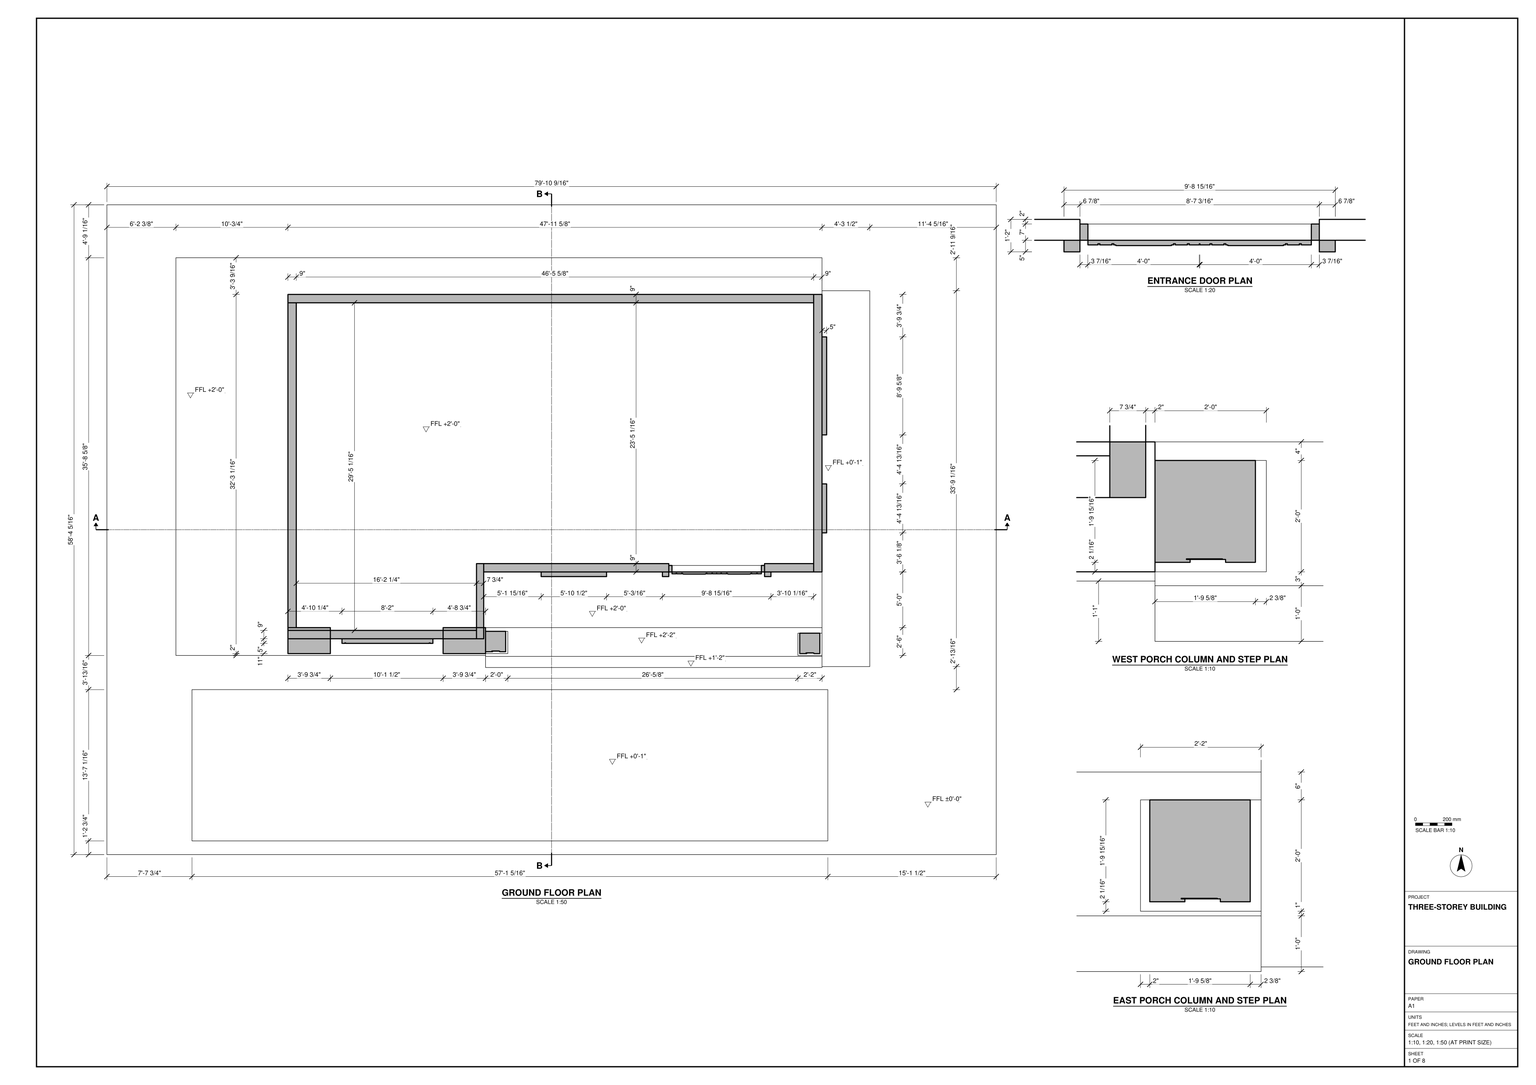
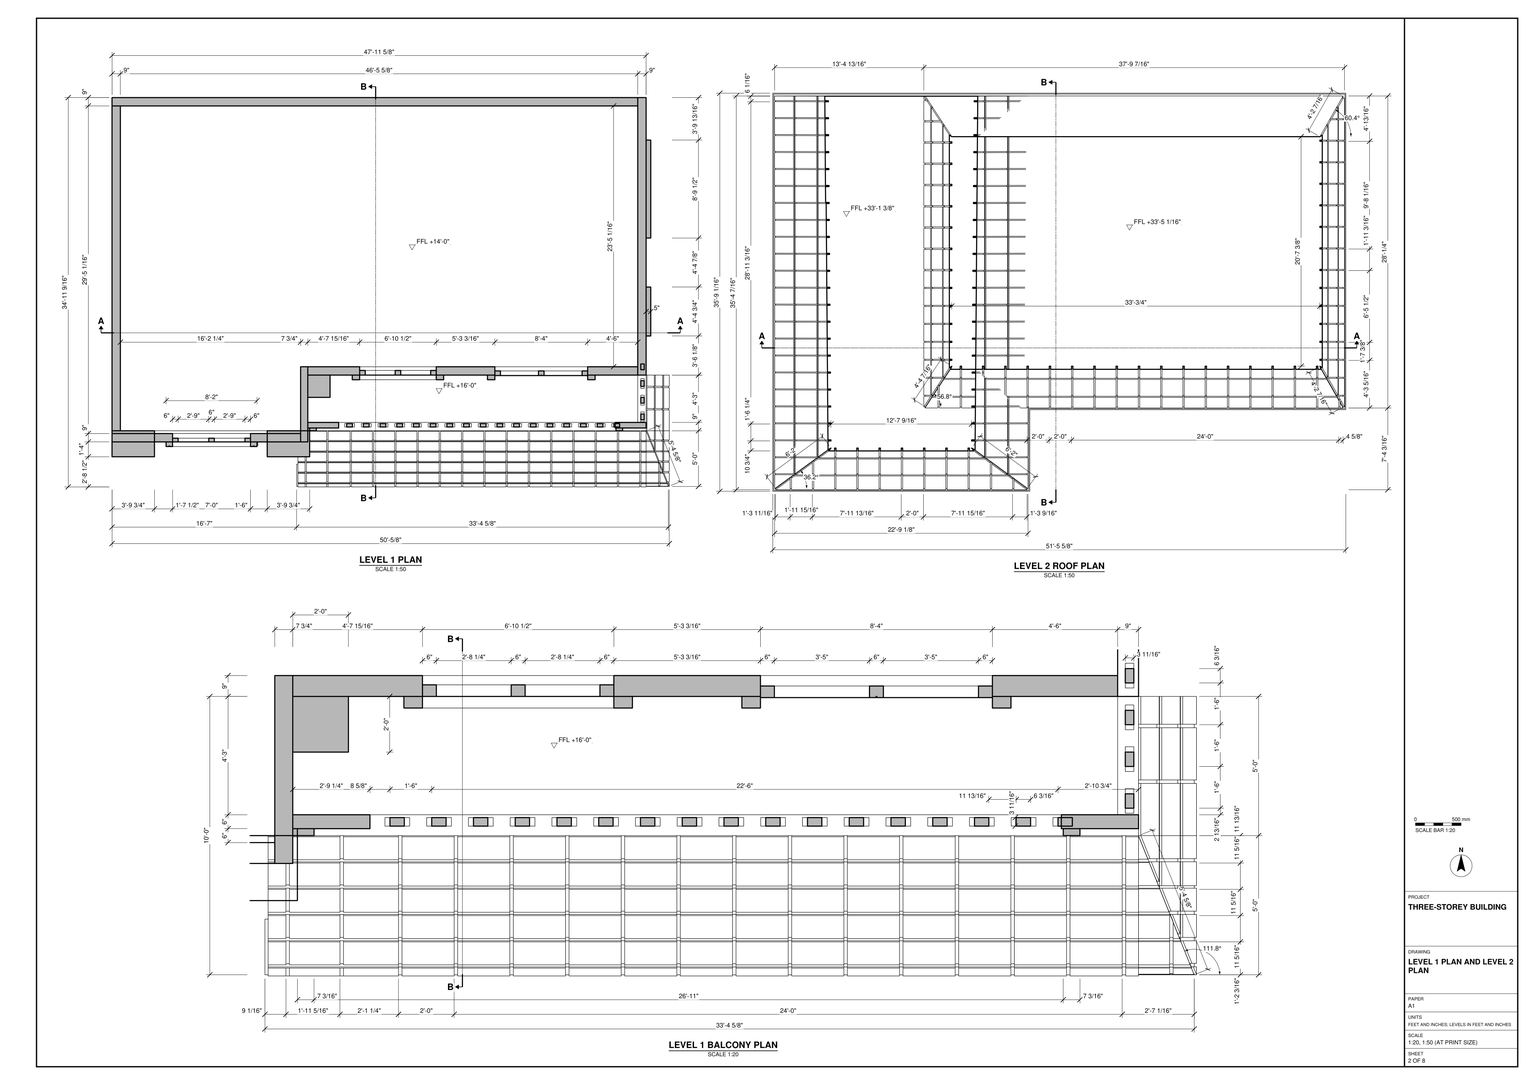
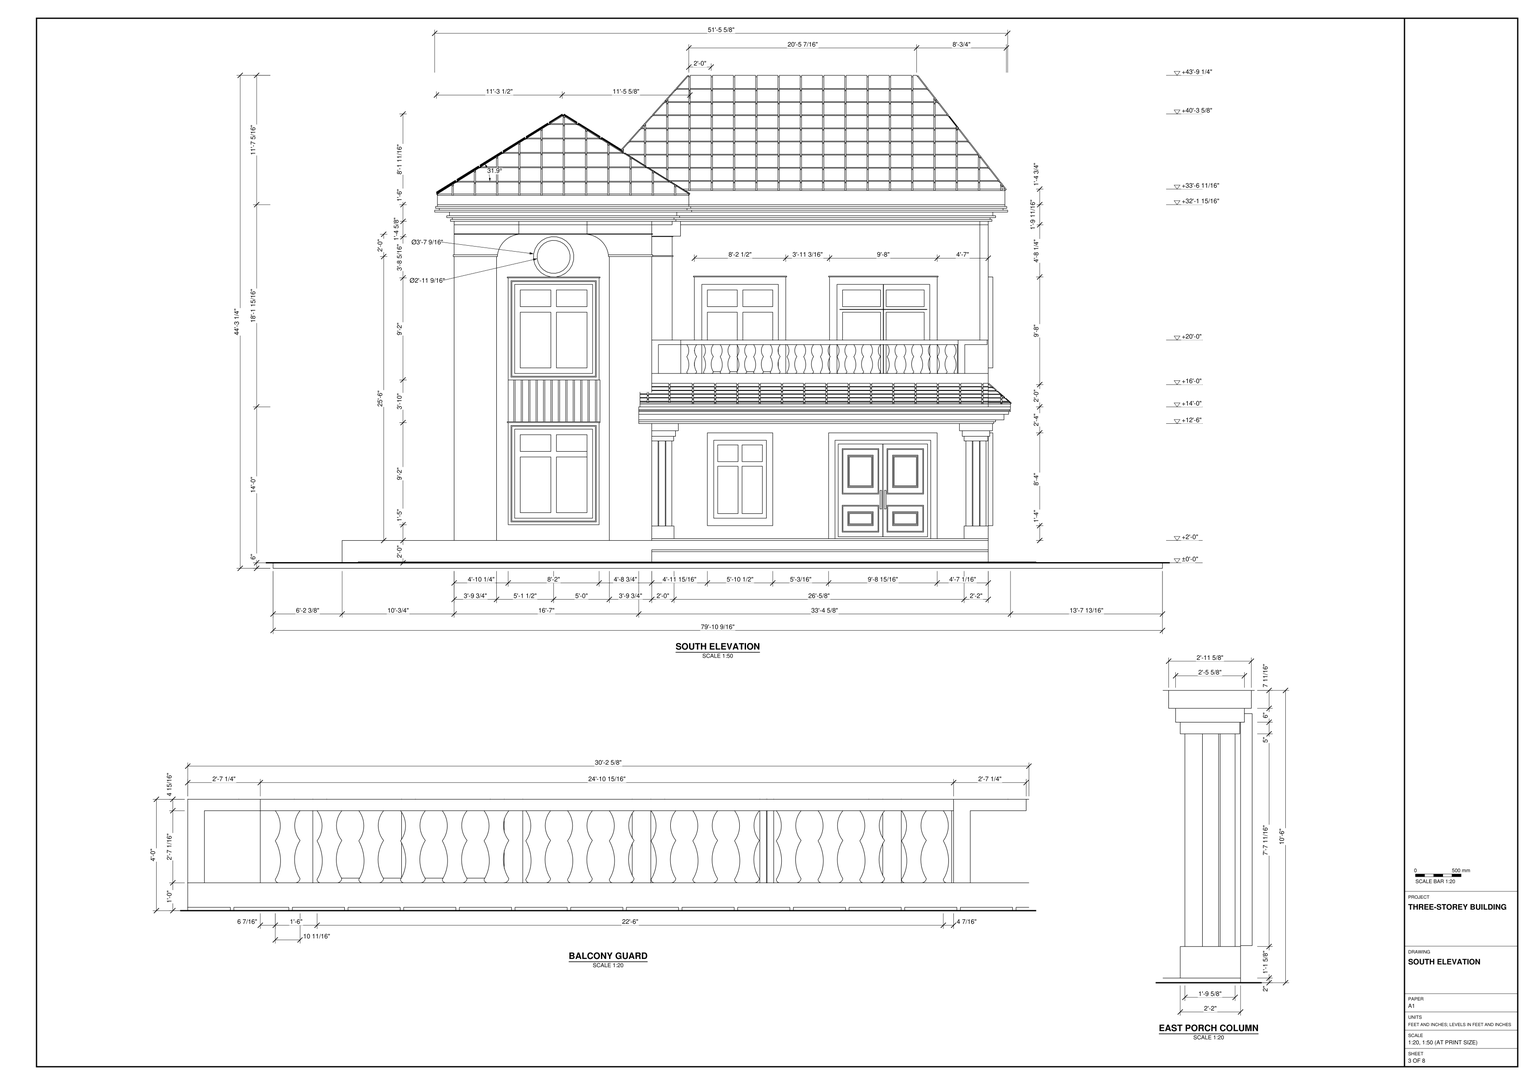
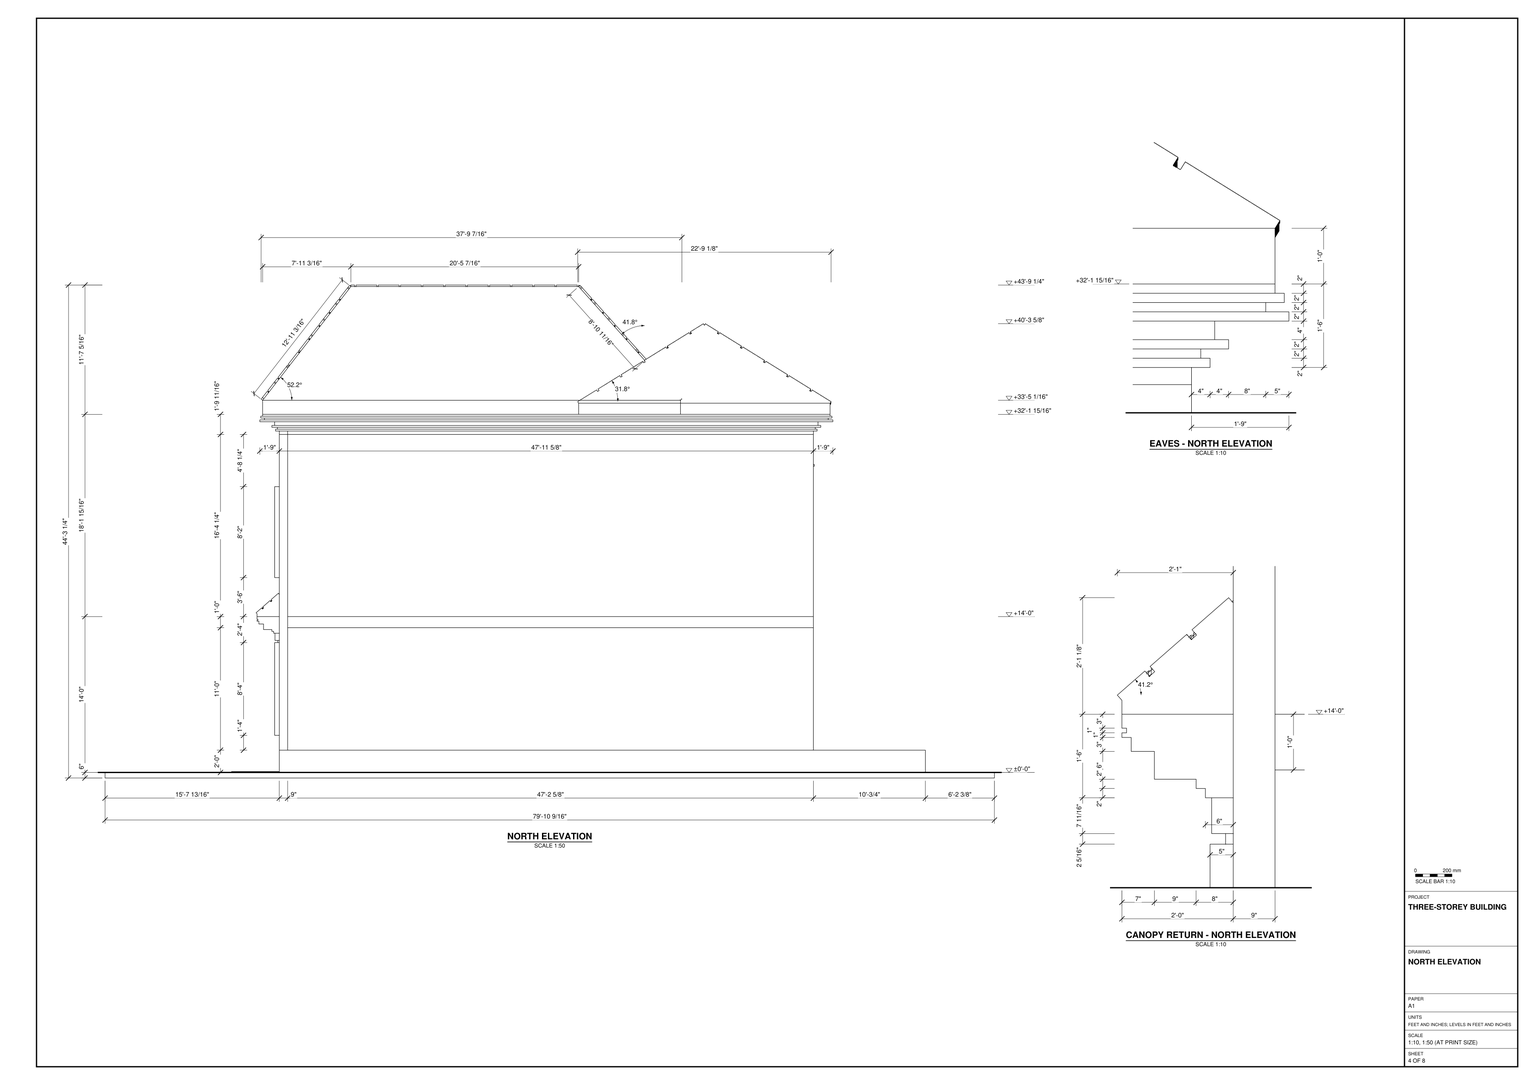
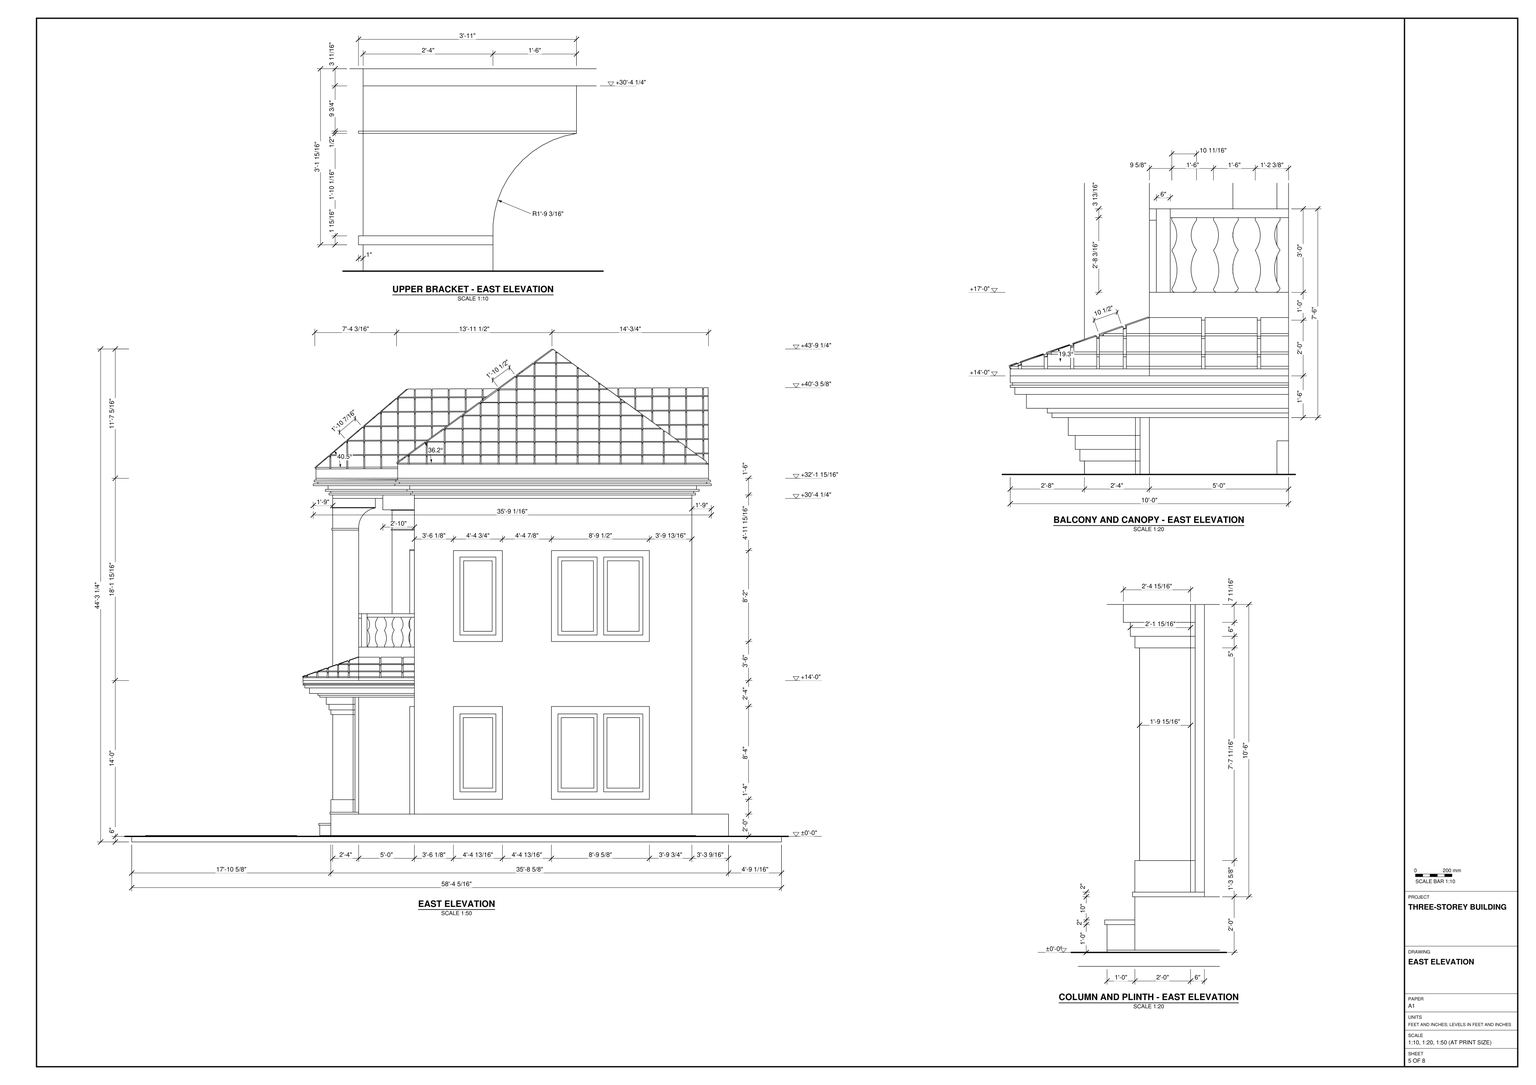
Build the three-storey building and its site base in SketchUp from task_files/diagram_01.pdf. Work in feet and inches. Including the base, the model must measure 79'-10 9/16" along X, 58'-4 5/16" along Y and 44'-3 1/4" along Z. Set the level references to ±0'-0", +14'-0" and +32'-1 15/16". Use the sections and elevations to distinguish these references from the raised entrance, balcony floor and roof ridges.

Lay out the walls at the thicknesses shown in plan, keeping the projecting west bay and the recessed entrance on the south side. Model the floor slabs, porch platform and entry steps. Set the paired entrance doors and divided window units into framed openings. On the projecting bay, align the windows vertically and include the ribbed panel between them and the circular feature above. Build the porch columns with their bases and stepped capitals. Above them, model the balcony floor, the sloping edge below its guard and the repeated balusters. Follow the roof plan for the intersecting pitched forms, and use the south elevation to set their different ridge heights and layered eaves.

Keep shell elements such as walls, slabs and roofs in separate groups or components. Keep each furniture or joinery piece shown separate, and use components for repeated parts. Decor and loose items, if shown, may be any suitable library components. Save one SketchUp model as output_files/three_storey_building_with_a_columned_porch_and_balcony.skp.

# SketchUp Ruby script. Lengths in inches.
U = 1.inch
M = Sketchup.active_model
def pt(a) = Geom::Point3d.new(a.map { |v| v * U })
def face(e, loops, mat)
  f = e.add_face(loops[0].map { |a| pt(a) })
  loops[1..].each { |l| e.add_face(l.map { |a| pt(a) }).erase! }
  f.material = f.back_material = mat if mat
  f
end
# faces: each face lists its corners as indices into pts; further lists are holes
def faces(e, pts, list, mat = nil) = list.each { |f| face(e, (f[0].is_a?(Array) ? f : [f]).map { |l| l.map { |i| pts[i] } }, mat) }
# xy, xz, yz: faces in a plane at the given z, y or x. An outline is a flat list of corners, or four numbers for a rectangle; further outlines are holes
def ring(l) = l.size == 4 ? [[l[0], l[1]], [l[2], l[1]], [l[2], l[3]], [l[0], l[3]]] : l.each_slice(2).to_a
def flat(e, list, mat, &to3) = list.each { |f| face(e, (f[0].is_a?(Array) ? f : [f]).map { |l| ring(l).map { |u, v| to3.(u, v) } }, mat) }
def xy(e, z, list, mat = nil) = flat(e, list, mat) { |x, y| [x, y, z] }
def xz(e, y, list, mat = nil) = flat(e, list, mat) { |x, z| [x, y, z] }
def yz(e, x, list, mat = nil) = flat(e, list, mat) { |y, z| [x, y, z] }
def lines(e, pts, list) = list.each { |a, b| e.add_line(pt(pts[a]), pt(pts[b])) }
# prism: a flat outline (further loops are holes) pulled along v
def prism(e, loops, v, mat = nil)
  f = face(e, loops, mat); d = Geom::Vector3d.new(v.map { |x| x * U })
  f.pushpull(f.normal.samedirection?(d) ? d.length : -d.length)
end
def box(e, o, s, mat = nil) = prism(e, [[o, [o[0] + s[0], o[1], o[2]], [o[0] + s[0], o[1] + s[1], o[2]], [o[0], o[1] + s[1], o[2]]]], [0, 0, s[2]], mat)
def at(x, y, z, deg = 0) = Geom::Transformation.translation(pt([x, y, z])) * Geom::Transformation.rotation(ORIGIN, Z_AXIS, deg.degrees)
def axes(o, x, y, z) = Geom::Transformation.new([*x, 0, *y, 0, *z, 0, *pt(o).to_a, 1])
def part(name) = M.definitions.add(name)
# library, detail: a bought-in or finely detailed component or shape, given as its bounding box
def library(name, o, s) = part(name).tap { |d| box(d.entities, o, s) }
def detail(e, o, s) = box(e.add_group.entities, o, s)
def put(e, d, t, mat = nil) = e.add_instance(d, t).tap { |i| i.material = mat if mat }
def group(e, t, mat = nil) = e.add_group.tap { |g| g.transformation = t; g.material = mat if mat }.entities
root = M.entities
M.materials.add("[Color C02]").color = [255, 204, 153]
M.materials.add("[Color D01]").color = [255, 242, 204]
M.materials.add("[Color M05]").color = [114, 114, 114]
M.materials.add("[Color M07]").color = [58, 58, 58]
M.materials.add("[Color M08]").color = [30, 30, 30]
M.materials.add("[Grass Dark Green]").color = [106, 157, 55]
M.materials.add("[Metal Rusted]").color = [184, 117, 91]
M.materials.add("[Translucent Glass Blue]").color = [100, 149, 237]
M.materials.add("[Translucent Glass Gray]").color = [128, 128, 128]
M.materials.add("[Translucent Glass Tinted]").color = [137, 125, 3]
c1 = library("Group\#7",[0,0,0],[1.375,98.4375,1.375])
c2 = library("Group\#12",[0,0,0],[1.375,35.875,1.375])
c3 = library("Group\#17",[0,-0.3,0],[112,2.3,100])
c4 = part("Group\#18")
prism(c4.entities,[[[0,2,20],[0,2,18.26],[0,0.74,18.26],[0,0.74,1.74],[0,2,1.74],[0,2,0],[0,0,0],[0,0,20]]],[1.99,0,0])
c5 = library("Group\#21",[0,0,0],[56,2,2])
c6 = library("Group\#22",[0,0,0],[2,2,18])
c7 = library("Group\#23",[0,0,0],[2,2,17.9375])
c8 = library("Group\#24",[0,0,0],[2,2,18])
c9 = library("Group\#25",[0,0,0],[2,2,18])
c10 = library("Group\#40",[-34.625,-0.5,0],[375.26,60.5,25.42])
c11 = library("Group\#41",[0,0,0],[24.99,60,25.13])
c12 = library("Group\#42",[0,0,0],[24,60,24.51])
c13 = library("Group\#43",[0,0,0],[24.99,60,25.13])
c14 = library("Group\#45",[0,0,0],[100,5,108])
c15 = library("Group\#46",[0,0,0],[88,2,2])
c16 = library("Group\#47",[0,0,0],[2,2,18])
c17 = library("Group\#48",[0,0,0],[1.99,1.99,18])
c18 = library("Group\#49",[0,0,0],[2,2,18])
c19 = library("Group\#50",[0,0,0],[1.99,1.99,18])
c20 = library("Group\#57",[0,0,0],[70.52,2,2])
c21 = library("Group\#58",[0,0,0],[2,2,18])
c22 = library("Group\#59",[0,0,0],[2,2,18])
c23 = library("Group\#60",[0,0,0],[2,2,18.0625])
c24 = library("Group\#61",[0,0,0],[1.99,1.99,18])
c25 = library("Group\#71",[0,0,0],[2,30.72,2])
c26 = library("Group\#73",[0,0,0],[1.625,83.52,1.625])
c27 = library("Group\#80",[0,0,0],[72,2,2])
c28 = library("Group\#81",[0,0,0],[1.99,1.99,18])
c29 = library("Group\#82",[0,0,0],[2,2,18])
c30 = library("Group\#83",[0,0,0],[2,2,18])
c31 = library("Group\#84",[0,0,0],[2,2,18])
c32 = library("Group\#91",[0,0,0],[72,2,2])
c33 = library("Group\#92",[0,0,0],[2,2,18])
c34 = library("Group\#93",[0,0,0],[2,2,18])
c35 = library("Group\#94",[0,0,0],[2,2,18])
c36 = library("Group\#95",[0,0,0],[2,2,18])
c37 = library("Group\#102",[0,-2,0],[99,4,45])
c38 = part("Group\#103")
box(c38.entities,[0,0,0],[45.74,28,306])
c39 = part("Group\#104")
box(c39.entities,[-1,-1,0],[47.74,29,1.9375])
c40 = library("Group\#106",[-24,0,0],[70.74,46,36])
c41 = library("Group\#107",[0,0,0],[43.33,5,43.33])
c42 = library("Group\#110",[0,-9,0],[33,34,175.9375])
c43 = library("Group\#113",[-1.05,-1.3,0],[273.09,424.42,99.7])
c44 = library("Group\#114",[-1.49,-1.18,0],[453.46,336.25,95.49])
c45 = part("Group\#116")
box(c45.entities,[0,0,0],[33.28,6,36])
c46 = part("Group\#117")
xy(c46.entities,0,[[0,0,7.19,3]])
xy(c46.entities,31.08,[[7.19,0,31.28,3]])
xy(c46.entities,36,[[0,0,7.19,3],[7.19,0,31.28,3]])
xz(c46.entities,0,[[0,0,7.19,0,7.19,31.08,31.28,31.08,31.28,36,0,36]])
xz(c46.entities,3,[[0,0,7.19,36],[7.19,31.08,31.28,36]])
yz(c46.entities,0,[[0,0,3,36]])
yz(c46.entities,7.19,[[0,0,3,31.08]])
yz(c46.entities,31.28,[[0,31.08,3,36]])
c47 = library("Group\#119",[0,0,0],[10.6875,3.6875,32.1875])
c48 = part("Group\#121")
xy(c48.entities,0,[[0,0,0,21.96,21.65,21.96,21.65,0,15.21,0,15.21,0.625,14.54,0.625,14.54,0.75,6.78,0.75,6.78,0.625,7.57,0.625,7.57,0],[6.78,0.625,14.54,0.75]])
xy(c48.entities,91.6875,[[0,0,7.57,0,7.57,0.625,6.78,0.625,6.78,0.75,14.54,0.75,14.54,0.625,15.21,0.625,15.21,0,21.65,0,21.65,21.96,0,21.96],[6.78,0.625,14.54,0.75]])
xz(c48.entities,0,[[0,0,7.57,91.6875],[15.21,0,21.65,91.6875]])
xz(c48.entities,0.625,[[6.78,0,7.57,91.6875],[7.57,0,14.54,91.6875],[14.54,0,15.21,91.6875]])
xz(c48.entities,0.75,[[6.78,0,14.54,91.6875]])
xz(c48.entities,21.96,[[0,0,21.65,91.6875]])
yz(c48.entities,0,[[0,0,21.96,91.6875]])
yz(c48.entities,6.78,[[0.625,0,0.75,91.6875]])
yz(c48.entities,7.57,[[0,0,0.625,91.6875]])
yz(c48.entities,14.54,[[0.625,0,0.75,91.6875]])
yz(c48.entities,15.21,[[0,0,0.625,91.6875]])
yz(c48.entities,21.65,[[0,0,21.96,91.6875]])
xy(root,387.9375,[[446.12,288.64,786.76,619.71]])
g1 = group(root,at(487.1875,390.1875,0))
box(g1,[-487.1875,-390.1875,0],[958.5625,700.3125,6])
g2 = group(root,at(530.76,403.26,6),"[Color D01]")
box(g2,[-456.375,-188.625,0],[696.375,428.625,24])
g3 = group(root,at(761.76,392.51,30),"[Color D01]")
prism(g3,[[[9,-87.87,0],[9,211.2,0],[9,211.2,343.9375],[9,-87.87,343.9375]],[[9,116.14,193],[9,116.14,277],[9,158.4,277],[9,158.4,193]],[[9,66.88,277],[9,109.14,277],[9,109.14,193],[9,66.88,193]],[[9,116.16,108],[9,158.4,108],[9,158.4,24],[9,116.16,24]],[[9,66.88,24],[9,66.88,108],[9,109.12,108],[9,109.12,24]],[[9,-38.72,277],[9,0,277],[9,0,193],[9,-38.72,193]],[[9,-38.72,24],[9,-38.72,108],[9,0,108],[9,0,24]]],[-9,0,0])
g4 = group(root,at(770.76,452.35,46),"[Color D01]")
prism(g4,[[[0,0,100],[0,105.6,100],[0,105.6,0],[0,0,0]],[[0,7.04,8],[0,49.28,8],[0,49.28,92],[0,7.04,92]],[[0,56.32,92],[0,56.32,8],[0,98.56,8],[0,98.56,92]]],[5,0,0])
g5 = group(root,at(767.76,459.39,54),"[Color M07]")
prism(g5,[[[3,0,0],[3,42.24,0],[3,42.24,84],[3,0,84]],[[3,38.72,80],[3,38.72,4],[3,3.52,4],[3,3.52,80]]],[-3,0,0])
g6 = group(root,at(767.76,508.67,54),"[Color M07]")
prism(g6,[[[3,0,84],[3,0,0],[3,42.24,0],[3,42.24,84]],[[3,3.52,80],[3,38.72,80],[3,38.72,4],[3,3.52,4]]],[-3,0,0])
put(root,c1,axes([768.57,462.91,126.73],[1,0,0],[0,0.88,0],[0,0,1]),"[Color M08]")
put(root,c1,axes([768.57,462.91,119.73],[1,0,0],[0,0.88,0],[0,0,1]),"[Color M08]")
put(root,c1,axes([768.57,462.91,112.73],[1,0,0],[0,0.88,0],[0,0,1]),"[Color M08]")
put(root,c1,axes([768.57,462.91,105.73],[1,0,0],[0,0.88,0],[0,0,1]),"[Color M08]")
put(root,c1,axes([768.57,462.91,98.73],[1,0,0],[0,0.88,0],[0,0,1]),"[Color M08]")
put(root,c1,axes([768.57,462.91,91.73],[1,0,0],[0,0.88,0],[0,0,1]),"[Color M08]")
put(root,c1,axes([768.57,462.91,84.73],[1,0,0],[0,0.88,0],[0,0,1]),"[Color M08]")
put(root,c1,axes([768.57,462.91,77.73],[1,0,0],[0,0.88,0],[0,0,1]),"[Color M08]")
put(root,c1,axes([768.57,462.91,70.73],[1,0,0],[0,0.88,0],[0,0,1]),"[Color M08]")
put(root,c1,axes([768.57,462.91,63.73],[1,0,0],[0,0.88,0],[0,0,1]),"[Color M08]")
g7 = group(root,at(770.76,512.19,58),"[Translucent Glass Gray]")
yz(g7,0,[[0,0,35.2,76]])
g8 = group(root,at(770.76,462.91,58),"[Translucent Glass Gray]")
yz(g8,0,[[0,0,35.2,76]])
g9 = group(root,at(770.76,346.75,46),"[Color D01]")
prism(g9,[[[5,0,0],[5,52.8,0],[5,52.8,100],[5,0,100]],[[5,7.04,8],[5,7.04,92],[5,45.76,92],[5,45.76,8]]],[-5,0,0])
g10 = group(root,at(767.76,353.79,54),"[Color M07]")
prism(g10,[[[0,0,84],[0,38.72,84],[0,38.72,0],[0,0,0]],[[0,3.52,80],[0,3.52,4],[0,35.2,4],[0,35.2,80]]],[3,0,0])
put(root,c2,axes([768.57,357.31,126.99],[1,0,0],[0,0.88,0],[0,0,1]),"[Color M08]")
put(root,c2,axes([768.57,357.31,119.99],[1,0,0],[0,0.88,0],[0,0,1]),"[Color M08]")
put(root,c2,axes([768.57,357.31,112.99],[1,0,0],[0,0.88,0],[0,0,1]),"[Color M08]")
put(root,c2,axes([768.57,357.31,105.99],[1,0,0],[0,0.88,0],[0,0,1]),"[Color M08]")
put(root,c2,axes([768.57,357.31,98.99],[1,0,0],[0,0.88,0],[0,0,1]),"[Translucent Glass Gray]")
put(root,c2,axes([768.57,357.31,91.99],[1,0,0],[0,0.88,0],[0,0,1]),"[Color M08]")
put(root,c2,axes([768.57,357.31,84.99],[1,0,0],[0,0.88,0],[0,0,1]),"[Color M08]")
put(root,c2,axes([768.57,357.31,77.99],[1,0,0],[0,0.88,0],[0,0,1]),"[Color M08]")
put(root,c2,axes([768.57,357.31,70.99],[1,0,0],[0,0.88,0],[0,0,1]),"[Color M08]")
put(root,c2,axes([768.57,357.31,63.99],[1,0,0],[0,0.88,0],[0,0,1]),"[Color M08]")
g11 = group(root,at(770.76,357.31,58),"[Translucent Glass Gray]")
yz(g11,0,[[0,0,31.68,76]])
g12 = group(root,at(564.36,304.64,30),"[Color D01]")
prism(g12,[[[-158.24,0,0],[41.28,0,0],[41.28,0,108],[144.48,0,108],[144.48,0,0],[197.4,0,0],[197.4,0,132],[-158.24,0,132]],[[-32.68,0,108],[-32.68,0,24],[-89.44,0,24],[-89.44,0,108]]],[0,9,0])
g13 = group(root,at(598.76,299.64,30),"[Color D01]")
prism(g13,[[[6.88,5,0],[0,5,0],[0,5,116],[116.96,5,116],[116.96,5,0],[110.08,5,0],[110.08,5,108],[6.88,5,108]]],[0,-5,0])
g14 = group(root,at(605.64,304.64,30),"[Color M07]")
prism(g14,[[[0,7,0],[0,7,108],[103.2,7,108],[103.2,7,0]],[[99.76,7,104],[3.44,7,104],[3.44,7,4],[99.76,7,4]]],[0,-7,0])
put(root,c3,axes([609.08,302.64,34],[0.86,0,0],[0,1,0],[0,0,1]),"[Color M07]")
put(root,c4,axes([654.23,300.64,64],[0.86,0,0],[0,1,0],[0,0,1]),"[Metal Rusted]")
put(root,c4,axes([658.91,300.64,64],[0.86,0,0],[0,1,0],[0,0,1]),"[Metal Rusted]")
g15 = group(root,at(457.72,299.64,46),"[Color D01]")
prism(g15,[[[80.84,0,100],[10.32,0,100],[10.32,0,0],[80.84,0,0]],[[73.96,0,92],[73.96,0,8],[17.2,0,8],[17.2,0,92]]],[0,5,0])
g16 = group(root,at(398.38,232.64,30),"[Color D01]")
box(g16,[0,0,0],[7.74,81,343.9375])
g17 = group(root,at(171.88,232.64,30),"[Color D01]")
xy(g17,0,[[23.25,0,226.5,9]])
xy(g17,24,[[88.5,0,172.5,9]])
xy(g17,120,[[88.5,0,172.5,9]])
xy(g17,180,[[88.5,0,172.5,9]])
xy(g17,276,[[88.5,0,172.5,9]])
xy(g17,330,[[23.25,-1,226.5,0],[23.25,0,226.5,9]])
xy(g17,330.5,[[23.25,-1,226.5,0],[23.25,0,226.5,9]])
xy(g17,343.9375,[[23.25,0,226.5,9]])
xz(g17,-1,[[23.25,330,226.5,330.5]])
xz(g17,0,[[[23.25,0,226.5,330],[88.5,24,172.5,120],[88.5,180,172.5,276]],[23.25,330.5,226.5,343.9375]])
xz(g17,9,[[[23.25,0,226.5,330],[88.5,24,172.5,120],[88.5,180,172.5,276]],[23.25,330,226.5,330.5],[23.25,330.5,226.5,343.9375]])
yz(g17,23.25,[[0,0,9,330],[-1,330,9,330.5],[0,330.5,9,343.9375]])
yz(g17,88.5,[[0,24,9,120],[0,180,9,276]])
yz(g17,172.5,[[0,24,9,120],[0,180,9,276]])
yz(g17,226.5,[[0,0,9,330],[-1,330,9,330.5],[0,330.5,9,343.9375]])
g18 = group(root,at(474.92,304.64,54),"[Color M07]")
prism(g18,[[[0,5,84],[56.76,5,84],[56.76,5,0],[0,5,0]],[[4.3,5,5],[26.23,5,5],[26.23,5,56],[4.3,5,56]],[[52.46,5,5],[52.46,5,56],[30.53,5,56],[30.53,5,5]],[[30.53,5,61],[52.46,5,61],[52.46,5,79],[30.53,5,79]],[[4.3,5,61],[26.23,5,61],[26.23,5,79],[4.3,5,79]]],[0,-5,0])
put(root,c5,axes([479.22,306.14,123],[0.86,0,0],[0,1,0],[0,0,1]),"[Color M08]")
put(root,c6,axes([519.86,306.14,115],[0.86,0,0],[0,1,0],[0,0,1]),"[Color M08]")
put(root,c7,axes([511.26,306.14,115],[0.86,0,0],[0,1,0],[0,0,1]),"[Color M08]")
put(root,c8,axes([493.63,306.14,115],[0.86,0,0],[0,1,0],[0,0,1]),"[Color M08]")
put(root,c9,axes([485.03,306.14,115],[0.86,0,0],[0,1,0],[0,0,1]),"[Color M08]")
g19 = group(root,at(479.22,304.64,115),"[Translucent Glass Tinted]")
xz(g19,0,[[0,0,21.93,18]])
g20 = group(root,at(505.45,304.64,115),"[Translucent Glass Tinted]")
xz(g20,0,[[0,0,21.93,18]])
g21 = group(root,at(479.22,304.64,59),"[Translucent Glass Tinted]")
xz(g21,0,[[0,0,21.93,51]])
g22 = group(root,at(505.45,304.64,59),"[Translucent Glass Tinted]")
xz(g22,0,[[0,0,21.93,51]])
g23 = group(root,at(83.39,594.71,30),"[Color D01]")
box(g23,[111.75,0,0],[566.625,9,132])
g24 = group(root,at(74.39,304.64,162),"[Color D01]")
prism(g24,[[[687.375,299.07,0],[687.375,0,0],[323.99,0,0],[323.99,-60,0],[120.75,-60,0],[120.75,299.07,0]]],[0,0,12])
g25 = group(root,at(406.12,208.64,156))
box(g25,[-7.74,0,0],[372.38,96,18])
g26 = group(root,at(394.12,184.64,156),"[Color C02]")
xy(g26,0,[[0,18,0,24,376.64,24,376.64,120,382.64,120,382.64,18]])
xy(g26,2,[[0,16,0,18,382.64,18,382.64,120,384.64,120,384.64,16]])
xy(g26,4,[[0,7,0,16,384.64,16,384.64,120,393.64,120,393.64,7]])
xy(g26,10,[[0,2,0,7,393.64,7,393.64,120,398.64,120,398.64,2]])
xy(g26,13,[[0,0,0,2,398.64,2,398.64,120,400.64,120,400.64,0]])
xy(g26,14,[[0,0,400.64,0,400.64,120,399.64,120,399.64,1,0,1]])
xy(g26,15,[[0,0,0,1,399.64,1,399.64,120,400.64,120,400.64,0]])
xy(g26,18,[[0,0,400.64,0,400.64,120,376.64,120,376.64,24,0,24]])
xz(g26,0,[[0,13,400.64,14],[0,15,400.64,18]])
xz(g26,1,[[0,14,399.64,15]])
xz(g26,2,[[0,10,398.64,13]])
xz(g26,7,[[0,4,393.64,10]])
xz(g26,16,[[0,2,384.64,4]])
xz(g26,18,[[0,0,382.64,2]])
xz(g26,24,[[0,0,376.64,9],[0,9,376.64,18]])
xz(g26,120,[[376.64,0,376.64,18,400.64,18,400.64,15,399.64,15,399.64,14,400.64,14,400.64,13,398.64,13,398.64,10,393.64,10,393.64,4,384.64,4,384.64,2,382.64,2,382.64,0]])
yz(g26,0,[[18,0,18,2,16,2,16,4,7,4,7,10,2,10,2,13,0,13,0,14,1,14,1,15,0,15,0,18,24,18,24,0]])
yz(g26,376.64,[[24,0,120,9],[24,9,120,18]])
yz(g26,382.64,[[18,0,120,2]])
yz(g26,384.64,[[16,2,120,4]])
yz(g26,393.64,[[7,4,120,10]])
yz(g26,398.64,[[2,10,120,13]])
yz(g26,399.64,[[1,14,120,15]])
yz(g26,400.64,[[0,13,120,14],[0,15,120,18]])
g27 = group(root,at(406.12,304.64,174),"[Color D01]")
prism(g27,[[[0,0,0],[355.64,0,0],[355.64,0,199.9375],[0,0,199.9375]],[[301.64,0,24],[201.64,0,24],[201.64,0,132],[301.64,0,132]],[[55.92,0,132],[138.44,0,132],[138.44,0,32],[55.92,0,32]]],[0,9,0])
g28 = group(root,at(430.12,244.64,174))
box(g28,[-24,0,0],[364.64,60,24])
put(root,c10,at(430.12,184.64,174),"[Color M05]")
put(root,c11,at(770.76,244.64,174),"[Color M05]")
put(root,c12,at(770.76,184.64,174),"[Color M05]")
put(root,c13,at(770.76,184.64,174),"[Color M05]")
g29 = group(root,at(599.76,299.64,198),"[Color D01]")
prism(g29,[[[0,0,0],[8,0,0],[8,0,108],[108,0,108],[108,0,0],[116,0,0],[116,0,116],[0,0,116]]],[0,5,0])
put(root,c14,at(607.76,304.14,198),"[Color M07]")
put(root,c15,at(613.76,305.64,290),"[Color M08]")
put(root,c16,at(625.26,305.64,282),"[Color M08]")
put(root,c17,at(641.27,305.64,282),"[Color M08]")
put(root,c18,at(672.26,305.64,282),"[Color M08]")
put(root,c19,at(688.27,305.64,282),"[Color M08]")
g30 = group(root,at(613.76,304.14,282),"[Translucent Glass Blue]")
xz(g30,0,[[0,0,41,18]])
g31 = group(root,at(660.76,304.14,282),"[Translucent Glass Blue]")
xz(g31,0,[[0,0,41,18]])
g32 = group(root,at(660.76,304.14,204),"[Translucent Glass Blue]")
xz(g32,0,[[0,0,41,72]])
g33 = group(root,at(613.76,304.14,204),"[Translucent Glass Blue]")
xz(g33,0,[[0,0,41,72]])
g34 = group(root,at(454.04,299.64,198),"[Color D01]")
prism(g34,[[[98.52,0,0],[98.52,0,116],[0,0,116],[0,0,0]],[[90.52,0,108],[90.52,0,8],[8,0,8],[8,0,108]]],[0,5,0])
g35 = group(root,at(462.04,304.64,206),"[Color M07]")
prism(g35,[[[82.52,5,0],[0,5,0],[0,5,100],[82.52,5,100]],[[6,5,6],[38.26,5,6],[38.26,5,70],[6,5,70]],[[44.26,5,70],[44.26,5,6],[76.52,5,6],[76.52,5,70]],[[6,5,76],[38.26,5,76],[38.26,5,94],[6,5,94]],[[44.26,5,76],[76.52,5,76],[76.52,5,94],[44.26,5,94]]],[0,-5,0])
put(root,c20,at(468.04,306.14,290),"[Color M08]")
put(root,c21,at(489.17,306.14,282),"[Color M08]")
put(root,c22,at(477.17,306.14,282),"[Color M08]")
put(root,c23,at(527.43,306.14,282),"[Color M08]")
put(root,c24,at(515.4375,306.14,282),"[Color M08]")
g36 = group(root,at(468.04,304.64,282),"[Translucent Glass Blue]")
xz(g36,0,[[0,0,32.26,18]])
g37 = group(root,at(506.3,304.64,282),"[Translucent Glass Blue]")
xz(g37,0,[[0,0,32.26,18]])
g38 = group(root,at(468.04,304.64,212),"[Translucent Glass Blue]")
xz(g38,0,[[0,0,32.26,64]])
g39 = group(root,at(506.3,304.64,212),"[Translucent Glass Blue]")
xz(g39,0,[[0,0,32.26,64]])
g40 = group(root,at(770.76,346.79,216),"[Color D01]")
prism(g40,[[[0,52.72,98],[0,52.72,0],[0,0,0],[0,0,98]],[[0,7,7],[0,45.72,7],[0,45.72,91],[0,7,91]]],[5,0,0])
g41 = group(root,at(766.76,353.79,223),"[Color M07]")
prism(g41,[[[0,0,84],[0,38.72,84],[0,38.72,0],[0,0,0]],[[0,4,4],[0,34.72,4],[0,34.72,80],[0,4,80]]],[4,0,0])
g42 = group(root,at(770.76,452.39,216),"[Color D01]")
prism(g42,[[[0,0,98],[0,105.52,98],[0,105.52,0],[0,0,0]],[[0,7,91],[0,7,7],[0,49.26,7],[0,49.26,91]],[[0,98.52,91],[0,56.26,91],[0,56.26,7],[0,98.52,7]]],[5,0,0])
g43 = group(root,at(766.76,459.39,223),"[Color M07]")
prism(g43,[[[0,0,84],[0,42.26,84],[0,42.26,0],[0,0,0]],[[0,38.26,4],[0,38.26,80],[0,4,80],[0,4,4]]],[4,0,0])
g44 = group(root,at(766.76,508.65,223),"[Color M07]")
prism(g44,[[[4,0,84],[4,0,0],[4,42.26,0],[4,42.26,84]],[[4,4,4],[4,4,80],[4,38.26,80],[4,38.26,4]]],[-4,0,0])
put(root,c25,at(767.76,357.79,296.39),"[Color M08]")
put(root,c25,at(767.76,357.79,289.39),"[Color M08]")
put(root,c25,at(767.76,357.79,282.39),"[Color M08]")
put(root,c25,at(767.76,357.79,275.39),"[Color M08]")
put(root,c25,at(767.76,357.79,268.39),"[Color M08]")
put(root,c25,at(767.76,357.79,261.39),"[Color M08]")
put(root,c25,at(767.76,357.79,254.39),"[Color M08]")
put(root,c25,at(767.76,357.79,247.39),"[Color M08]")
put(root,c25,at(767.76,357.79,240.39),"[Color M08]")
put(root,c25,at(767.76,357.79,233.39),"[Color M08]")
g45 = group(root,at(770.76,357.79,227),"[Translucent Glass Gray]")
yz(g45,0,[[0,0,30.72,76]])
put(root,c26,at(767.95,463.39,295.02),"[Color M08]")
put(root,c26,at(767.95,463.39,288.02),"[Color M08]")
put(root,c26,at(767.95,463.39,281.02),"[Color M08]")
put(root,c26,at(767.95,463.39,274.02),"[Color M08]")
put(root,c26,at(767.95,463.39,267.02),"[Color M08]")
put(root,c26,at(767.95,463.39,260.02),"[Color M08]")
put(root,c26,at(767.95,463.39,253.02),"[Color M08]")
put(root,c26,at(767.95,463.39,246.02),"[Color M08]")
put(root,c26,at(767.95,463.39,239.02),"[Color M08]")
put(root,c26,at(767.95,463.39,232.02),"[Color M08]")
g46 = group(root,at(770.76,512.65,227),"[Translucent Glass Gray]")
yz(g46,0,[[0,0,34.26,76]])
g47 = group(root,at(770.76,463.39,227),"[Translucent Glass Gray]")
yz(g47,0,[[0,0,34.26,76]])
g48 = group(root,at(598.76,299.64,314))
box(g48,[0,0,0],[118,5,1])
g49 = group(root,at(453.04,299.64,314))
box(g49,[0,0,0],[100.52,5,1])
g50 = group(root,at(253.38,227.64,47),"[Color C02]")
xy(g50,0,[[0,0,98,5]])
xy(g50,3,[[3,0,95,0.5]])
xy(g50,4,[[4,0,94,0.5]])
xy(g50,7,[[7,0,91,5]])
xy(g50,103,[[7,0,91,5]])
xy(g50,106,[[4,0,94,0.5]])
xy(g50,107,[[3,0,95,0.5]])
xy(g50,110,[[0,0,98,5]])
xz(g50,0,[[[0,0,98,110],[3,3,95,107]],[[4,4,94,106],[7,7,91,103]]])
xz(g50,0.5,[[[3,3,95,107],[4,4,94,106]]])
xz(g50,5,[[[0,0,98,110],[7,7,91,103]]])
yz(g50,0,[[0,0,5,110]])
yz(g50,3,[[0,3,0.5,107]])
yz(g50,4,[[0,4,0.5,106]])
yz(g50,7,[[0,7,5,103]])
yz(g50,91,[[0,7,5,103]])
yz(g50,94,[[0,4,0.5,106]])
yz(g50,95,[[0,3,0.5,107]])
yz(g50,98,[[0,0,5,110]])
g51 = group(root,at(260.38,232.64,54),"[Color M07]")
xy(g51,0,[[0,0,84,4]])
xy(g51,6,[[6,0,39,4],[45,0,78,4]])
xy(g51,66,[[6,0,39,4],[45,0,78,4]])
xy(g51,72,[[6,0,39,4],[45,0,78,4]])
xy(g51,90,[[6,0,39,4],[45,0,78,4]])
xy(g51,96,[[0,0,84,4]])
xz(g51,0,[[[0,0,84,96],[45,6,45,66,78,66,78,72,45,72,45,90,78,90,78,6],[6,6,39,66],[6,72,39,90]]])
xz(g51,4,[[[0,0,84,96],[45,6,78,6,78,90,45,90,45,72,78,72,78,66,45,66],[6,6,39,66],[6,72,39,90]]])
yz(g51,0,[[0,0,4,96]])
yz(g51,6,[[0,6,4,66],[0,72,4,90]])
yz(g51,39,[[0,6,4,66],[0,72,4,90]])
yz(g51,45,[[0,6,4,66],[0,72,4,90]])
yz(g51,78,[[0,6,4,66],[0,66,4,72],[0,72,4,90]])
yz(g51,84,[[0,0,4,96]])
put(root,c27,at(266.38,233.64,134),"[Color M08]")
put(root,c28,at(275.89,233.64,126),"[Color M08]")
put(root,c29,at(287.88,233.64,126),"[Color M08]")
put(root,c30,at(314.88,233.64,126),"[Color M08]")
put(root,c31,at(326.88,233.64,126),"[Color M08]")
g52 = group(root,at(266.38,232.64,126),"[Translucent Glass Tinted]")
xz(g52,0,[[0,0,33,18]])
g53 = group(root,at(305.38,232.64,126),"[Translucent Glass Tinted]")
xz(g53,0,[[0,0,33,18]])
g54 = group(root,at(305.38,232.64,60),"[Translucent Glass Tinted]")
xz(g54,0,[[0,0,33,60]])
g55 = group(root,at(266.38,232.64,60),"[Translucent Glass Tinted]")
xz(g55,0,[[0,0,33,60]])
g56 = group(root,at(253.38,227.64,203),"[Color C02]")
xy(g56,0,[[0,0,98,5]])
xy(g56,3.02,[[3.02,0,94.98,0.5]])
xy(g56,4.02,[[4.02,0,93.98,0.5]])
xy(g56,7,[[7,0,91,5]])
xy(g56,103,[[7,0,91,5]])
xy(g56,105.98,[[4.02,0,93.98,0.5]])
xy(g56,106.98,[[3.02,0,94.98,0.5]])
xy(g56,110,[[0,0,98,5]])
xz(g56,0,[[[0,0,98,110],[3.02,3.02,94.98,106.98]],[[4.02,4.02,93.98,105.98],[7,7,91,103]]])
xz(g56,0.5,[[[3.02,3.02,94.98,106.98],[4.02,4.02,93.98,105.98]]])
xz(g56,5,[[[0,0,98,110],[7,7,91,103]]])
yz(g56,0,[[0,0,5,110]])
yz(g56,3.02,[[0,3.02,0.5,106.98]])
yz(g56,4.02,[[0,4.02,0.5,105.98]])
yz(g56,7,[[0,7,5,103]])
yz(g56,91,[[0,7,5,103]])
yz(g56,93.98,[[0,4.02,0.5,105.98]])
yz(g56,94.98,[[0,3.02,0.5,106.98]])
yz(g56,98,[[0,0,5,110]])
g57 = group(root,at(260.38,232.64,210),"[Color M07]")
prism(g57,[[[0,0,96],[0,0,0],[84,0,0],[84,0,96]],[[6,0,66],[39,0,66],[39,0,6],[6,0,6]],[[78,0,66],[78,0,6],[45,0,6],[45,0,66]],[[78,0,72],[45,0,72],[45,0,90],[78,0,90]],[[6,0,72],[6,0,90],[39,0,90],[39,0,72]]],[0,4,0])
put(root,c32,at(266.38,233.64,290),"[Color M08]")
put(root,c33,at(275.88,233.64,282),"[Color M08]")
put(root,c34,at(287.88,233.64,282),"[Color M08]")
put(root,c35,at(314.88,233.64,282),"[Color M08]")
put(root,c36,at(326.88,233.64,282),"[Color M08]")
g58 = group(root,at(266.38,232.64,282),"[Translucent Glass Blue]")
xz(g58,0,[[0,0,33,18]])
g59 = group(root,at(305.38,232.64,282),"[Translucent Glass Blue]")
xz(g59,0,[[0,0,33,18]])
g60 = group(root,at(266.38,232.64,216),"[Translucent Glass Blue]")
xz(g60,0,[[0,0,33,60]])
g61 = group(root,at(305.38,232.64,216),"[Translucent Glass Blue]")
xz(g61,0,[[0,0,33,60]])
g62 = group(root,at(252.38,227.64,157))
box(g62,[0,0,0],[100,5,1])
g63 = group(root,at(252.38,227.64,313))
box(g63,[0,0,0],[100,5,1])
put(root,c37,at(253.38,230.64,158),"[Color D01]")
put(root,c38,at(362.38,216.64,30),"[Color D01]")
put(root,c39,at(362.38,216.64,336))
put(root,c40,at(362.38,216.64,337.9375),"[Color D01]")
put(root,c39,at(195.13,216.64,336))
g64 = group(root,at(195.13,216.64,337.9375),"[Color D01]")
box(g64,[143.25,-1,22.0625],[70.74,1,0.5])
detail(g64,[0,-1,0],[69.74,29,36])
put(root,c38,at(195.13,216.64,30),"[Color D01]")
put(root,c41,at(280.72,227.64,314),"[Translucent Glass Gray]")
g65 = group(root,at(195.13,244.64,30),"[Color D01]")
box(g65,[0,0,0],[9,350.07,132])
g66 = group(root,at(195.13,594.71,174),"[Color D01]")
box(g66,[0,0,0],[566.63,9,199.9375])
g67 = group(root,at(195.13,244.64,174),"[Color D01]")
box(g67,[0,0,0],[9,350.07,199.9375])
put(root,c42,at(406.12,279.64,198),"[Color D01]")
g68 = group(root,at(195.13,216.64,373.9375),"[Color C02]")
prism(g68,[[[575.63,88,-3.6875],[234.99,88,-3.6875],[234.99,0,-3.6875],[0,0,-3.6875],[0,387.07,-3.6875],[575.63,387.07,-3.6875]]],[0,0,21.6875])
g69 = group(root,at(174.13,195.64,373.9375),"[Color C02]")
xy(g69,0,[[[17,17,17,412.07,600.63,412.07,600.63,105,259.99,105,259.99,17],[21,21,255.99,21,255.99,109,596.63,109,596.63,408.07,21,408.07]]])
xy(g69,2,[[[17,17,259.99,17,259.99,105,600.63,105,600.63,412.07,17,412.07],[19,19,19,410.07,598.63,410.07,598.63,107,257.99,107,257.99,19]]])
xy(g69,4,[[[13,13,13,416.07,604.63,416.07,604.63,101,263.99,101,263.99,13],[19,19,257.99,19,257.99,107,598.63,107,598.63,410.07,19,410.07]]])
xy(g69,6,[[[13,13,263.99,13,263.99,101,604.63,101,604.63,416.07,13,416.07],[16,16,16,413.07,601.63,413.07,601.63,104,260.99,104,260.99,16]]])
xy(g69,9,[[21,21,21,408.07,596.63,408.07,596.63,109,255.99,109,255.99,21]])
xy(g69,10,[[[0,0,0,429.07,617.63,429.07,617.63,88,276.99,88,276.99,0],[16,16,260.99,16,260.99,104,601.63,104,601.63,413.07,16,413.07]]])
xy(g69,12,[[[0,0,276.99,0,276.99,88,617.63,88,617.63,429.07,0,429.07],[5,5,5,424.07,612.63,424.07,612.63,93,271.99,93,271.99,5]]])
xy(g69,14,[[[1,1,1,428.07,616.63,428.07,616.63,89,275.99,89,275.99,1],[5,5,271.99,5,271.99,93,612.63,93,612.63,424.07,5,424.07]]])
xy(g69,16,[[[1,1,275.99,1,275.99,89,616.63,89,616.63,428.07,1,428.07],[3,3,3,426.07,614.63,426.07,614.63,91,273.99,91,273.99,3]]])
xy(g69,18,[[[3,3,273.99,3,273.99,91,614.63,91,614.63,426.07,3,426.07],[21,21,21,408.07,596.63,408.07,596.63,109,255.99,109,255.99,21]]])
xz(g69,0,[[0,10,276.99,12]])
xz(g69,1,[[1,14,275.99,16]])
xz(g69,3,[[3,16,273.99,18]])
xz(g69,5,[[5,12,271.99,14]])
xz(g69,13,[[13,4,263.99,6]])
xz(g69,16,[[16,6,260.99,10]])
xz(g69,17,[[17,0,259.99,2]])
xz(g69,19,[[19,2,257.99,4]])
xz(g69,21,[[21,0,255.99,9],[21,9,255.99,18]])
xz(g69,88,[[276.99,10,617.63,12]])
xz(g69,89,[[275.99,14,616.63,16]])
xz(g69,91,[[273.99,16,614.63,18]])
xz(g69,93,[[271.99,12,612.63,14]])
xz(g69,101,[[263.99,4,604.63,6]])
xz(g69,104,[[260.99,6,601.63,10]])
xz(g69,105,[[259.99,0,600.63,2]])
xz(g69,107,[[257.99,2,598.63,4]])
xz(g69,109,[[255.99,0,596.63,9],[255.99,9,596.63,18]])
xz(g69,408.07,[[21,0,596.63,9],[21,9,596.63,18]])
xz(g69,410.07,[[19,2,598.63,4]])
xz(g69,412.07,[[17,0,600.63,2]])
xz(g69,413.07,[[16,6,601.63,10]])
xz(g69,416.07,[[13,4,604.63,6]])
xz(g69,424.07,[[5,12,612.63,14]])
xz(g69,426.07,[[3,16,614.63,18]])
xz(g69,428.07,[[1,14,616.63,16]])
xz(g69,429.07,[[0,10,617.63,12]])
yz(g69,0,[[0,10,429.07,12]])
yz(g69,1,[[1,14,428.07,16]])
yz(g69,3,[[3,16,426.07,18]])
yz(g69,5,[[5,12,424.07,14]])
yz(g69,13,[[13,4,416.07,6]])
yz(g69,16,[[16,6,413.07,10]])
yz(g69,17,[[17,0,412.07,2]])
yz(g69,19,[[19,2,410.07,4]])
yz(g69,21,[[21,0,408.07,9],[21,9,408.07,18]])
yz(g69,255.99,[[21,0,109,9],[21,9,109,18]])
yz(g69,257.99,[[19,2,107,4]])
yz(g69,259.99,[[17,0,105,2]])
yz(g69,260.99,[[16,6,104,10]])
yz(g69,263.99,[[13,4,101,6]])
yz(g69,271.99,[[5,12,93,14]])
yz(g69,273.99,[[3,16,91,18]])
yz(g69,275.99,[[1,14,89,16]])
yz(g69,276.99,[[0,10,88,12]])
yz(g69,596.63,[[109,0,408.07,9],[109,9,408.07,18]])
yz(g69,598.63,[[107,2,410.07,4]])
yz(g69,600.63,[[105,0,412.07,2]])
yz(g69,601.63,[[104,6,413.07,10]])
yz(g69,604.63,[[101,4,416.07,6]])
yz(g69,612.63,[[93,12,424.07,14]])
yz(g69,614.63,[[91,16,426.07,18]])
yz(g69,616.63,[[89,14,428.07,16]])
yz(g69,617.63,[[88,10,429.07,12]])
put(root,c43,at(177.13,198.58,389.9375),"[Color M05]")
put(root,c44,axes([338.37,286.64,391.9375],[1,0,0],[0,1,0],[0,0,1.4592]),"[Color M05]")
g70 = group(root,at(406.12,244.64,198),"[Color C02]")
prism(g70,[[[0,0,0],[0,9,0],[355.64,9,0],[355.64,60,0],[364.64,60,0],[364.64,0,0]]],[0,0,12])
put(root,c45,at(406.12,247.64,210),"[Color D01]")
put(root,c46,at(408.12,244.64,210),"[Color C02]")
put(root,c45,at(737.48,247.64,210),"[Color D01]")
put(root,c46,at(738.31,244.64,210),"[Color C02]")
g71 = group(root,at(439.4,244.64,241.08),"[Color C02]")
box(g71,[0,0,0],[298.91,9,4.92])
put(root,c47,at(445.87,248.72,210),"[Color D01]")
put(root,c47,at(463.87,248.72,210),"[Color D01]")
put(root,c47,at(481.87,248.72,210),"[Color D01]")
put(root,c47,at(499.87,248.72,210),"[Color D01]")
put(root,c47,at(517.87,248.72,210),"[Color D01]")
put(root,c47,at(535.87,248.72,210),"[Color D01]")
put(root,c47,at(553.87,248.72,210),"[Color D01]")
put(root,c47,at(571.87,248.72,210),"[Color D01]")
put(root,c47,at(589.87,248.72,210),"[Color D01]")
put(root,c47,at(607.87,248.72,210),"[Color D01]")
put(root,c47,at(625.87,248.72,210),"[Color D01]")
put(root,c47,at(643.87,248.72,210),"[Color D01]")
put(root,c47,at(661.87,248.72,210),"[Color D01]")
put(root,c47,at(679.87,248.72,210),"[Color D01]")
put(root,c47,at(697.87,248.72,210),"[Color D01]")
put(root,c47,at(715.87,248.72,210),"[Color D01]")
put(root,c47,at(733.87,248.72,210),"[Color D01]")
put(root,c47,at(768.73,254.28,210,90),"[Color D01]")
put(root,c47,at(768.73,272.28,210,90),"[Color D01]")
put(root,c47,at(768.73,290.28,210,90),"[Color D01]")
put(root,c47,at(768.73,308.28,210,90))
g72 = group(root,at(763.51,253.64,242),"[Color C02]")
box(g72,[0,0,0.1875],[7.25,51,3.8125])
g73 = group(root,at(746.76,209.67,148.29),"[Color D01]")
box(g73,[-7,0,0],[35.65,28.96,7.71])
g74 = group(root,at(746.76,214.64,30),"[Color D01]")
box(g74,[-2,0,2],[26,24,13.6])
put(root,c48,at(746.76,216.67,45.6),"[Color D01]")
g75 = group(root,at(746.76,212.67,142.29),"[Color D01]")
box(g75,[-4,0,0],[29.65,25.96,6])
g76 = group(root,at(746.76,214.67,137.29),"[Color D01]")
box(g76,[-2,0,0],[25.65,23.96,5])
g77 = group(root,at(408.12,202.64,6),"[Color D01]")
box(g77,[0,0,0],[362.64,12,12])
g78 = group(root,at(408.12,201.64,18),"[Color D01]")
box(g78,[0,0,0],[362.64,13,2])
g79 = group(root,at(408.12,216.64,30),"[Color D01]")
box(g79,[0,0,2],[24,24,13.6])
g80 = group(root,at(408.12,214.67,142.29),"[Color D01]")
box(g80,[0,0,0],[25.65,25.96,6])
g81 = group(root,at(408.12,211.67,148.29),"[Color D01]")
box(g81,[0,0,0],[28.65,28.96,7.71])
g82 = group(root,at(408.12,216.67,137.29),"[Color D01]")
box(g82,[0,0,0],[23.65,23.96,5])
put(root,c48,at(408.12,218.67,45.6),"[Color D01]")
g83 = group(root,at(408.12,214.64,30),"[Color D01]")
box(g83,[0,-1,0],[362.64,31,2])
g84 = group(root,at(770.76,202.64,6))
xy(g84,0,[[0,0,51.5,405.0625]])
xy(g84,1,[[0,0,51.5,405.0625]],"[Grass Dark Green]")
xz(g84,0,[[0,0,51.5,1]])
xz(g84,405.0625,[[0,0,51.5,1]])
yz(g84,0,[[0,0,405.0625,1]])
yz(g84,51.5,[[0,0,405.0625,1]])
g85 = group(root,at(91.73,14.76,6))
xy(g85,0,[[0,0,685.3125,163.0625]])
xy(g85,1,[[0,0,685.3125,163.0625]],"[Grass Dark Green]")
xz(g85,0,[[0,0,685.3125,1]])
xz(g85,163.0625,[[0,0,685.3125,1]])
yz(g85,0,[[0,0,163.0625,1]])
yz(g85,685.3125,[[0,0,163.0625,1]])
